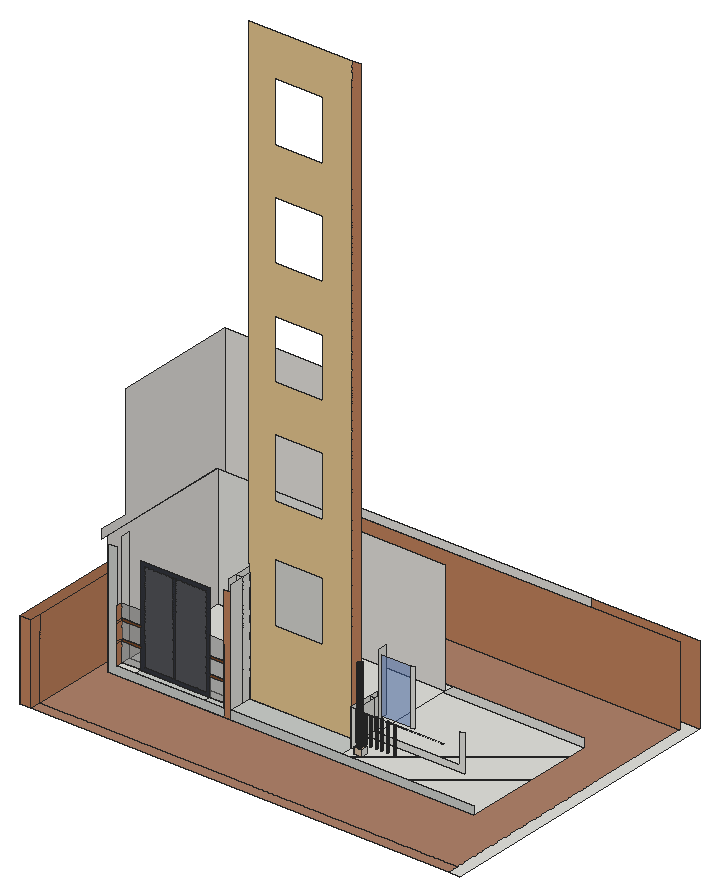
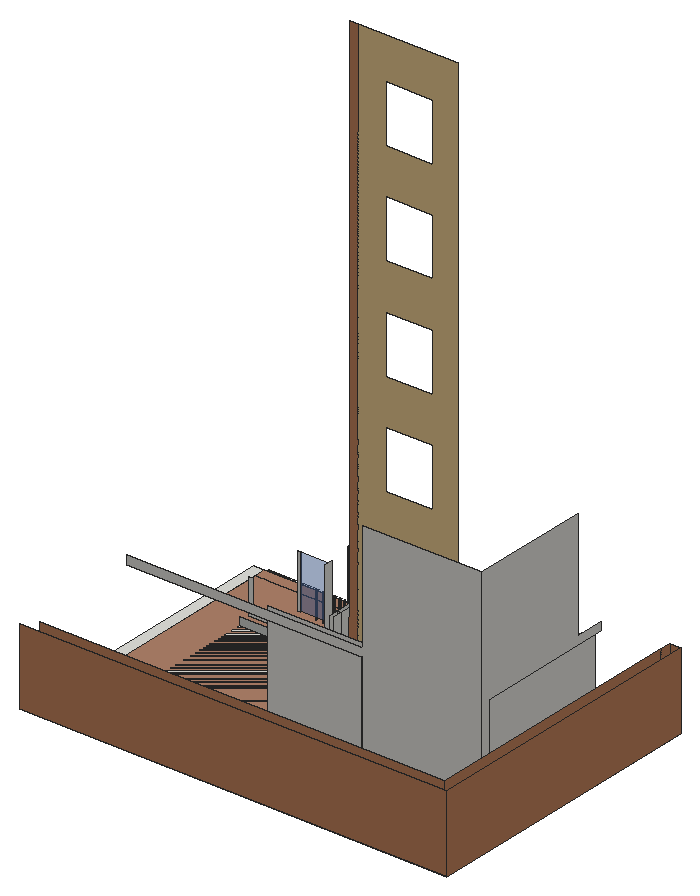
# SketchUp Ruby script. Lengths in inches.
U = 1.inch
M = Sketchup.active_model
def pt(a) = Geom::Point3d.new(a.map { |v| v * U })
def face(e, loops, mat)
  f = e.add_face(loops[0].map { |a| pt(a) })
  loops[1..].each { |l| e.add_face(l.map { |a| pt(a) }).erase! }
  f.material = f.back_material = mat if mat
  f
end
# faces: each face lists its corners as indices into pts; further lists are holes
def faces(e, pts, list, mat = nil) = list.each { |f| face(e, (f[0].is_a?(Array) ? f : [f]).map { |l| l.map { |i| pts[i] } }, mat) }
# xy, xz, yz: faces in a plane at the given z, y or x. An outline is a flat list of corners, or four numbers for a rectangle; further outlines are holes
def ring(l) = l.size == 4 ? [[l[0], l[1]], [l[2], l[1]], [l[2], l[3]], [l[0], l[3]]] : l.each_slice(2).to_a
def flat(e, list, mat, &to3) = list.each { |f| face(e, (f[0].is_a?(Array) ? f : [f]).map { |l| ring(l).map { |u, v| to3.(u, v) } }, mat) }
def xy(e, z, list, mat = nil) = flat(e, list, mat) { |x, y| [x, y, z] }
def xz(e, y, list, mat = nil) = flat(e, list, mat) { |x, z| [x, y, z] }
def yz(e, x, list, mat = nil) = flat(e, list, mat) { |y, z| [x, y, z] }
def lines(e, pts, list) = list.each { |a, b| e.add_line(pt(pts[a]), pt(pts[b])) }
# prism: a flat outline (further loops are holes) pulled along v
def prism(e, loops, v, mat = nil)
  f = face(e, loops, mat); d = Geom::Vector3d.new(v.map { |x| x * U })
  f.pushpull(f.normal.samedirection?(d) ? d.length : -d.length)
end
def box(e, o, s, mat = nil) = prism(e, [[o, [o[0] + s[0], o[1], o[2]], [o[0] + s[0], o[1] + s[1], o[2]], [o[0], o[1] + s[1], o[2]]]], [0, 0, s[2]], mat)
def at(x, y, z, deg = 0) = Geom::Transformation.translation(pt([x, y, z])) * Geom::Transformation.rotation(ORIGIN, Z_AXIS, deg.degrees)
def axes(o, x, y, z) = Geom::Transformation.new([*x, 0, *y, 0, *z, 0, *pt(o).to_a, 1])
def part(name) = M.definitions.add(name)
# library, detail: a bought-in or finely detailed component or shape, given as its bounding box
def library(name, o, s) = part(name).tap { |d| box(d.entities, o, s) }
def detail(e, o, s) = box(e.add_group.entities, o, s)
def put(e, d, t, mat = nil) = e.add_instance(d, t).tap { |i| i.material = mat if mat }
def group(e, t, mat = nil) = e.add_group.tap { |g| g.transformation = t; g.material = mat if mat }.entities
root = M.entities
M.materials.add("[Basic Tile]").color = [203, 206, 202]
M.materials.add("[Blinds Roman Hobbled Blue]").color = [81, 82, 87]
M.materials.add("[Formica Laminate Dark]").color = [50, 53, 60]
M.materials.add("[Formica Laminate Light]").color = [213, 189, 164]
M.materials.add("[Formica Speckled Grey]").color = [112, 125, 132]
M.materials.add("[Pavers Driveway Brick]").color = [176, 130, 106]
M.materials.add("[Stone Sandstone Ashlar Light]").color = [226, 196, 141]
M.materials.add("[Terrazzo Tile Accent]").color = [224, 221, 217]
M.materials.add("[Translucent Glass Blue]").color = [85, 126, 201]
M.materials["[Translucent Glass Blue]"].alpha = 0.5
M.materials.add("[Translucent Glass Gray]").color = [128, 128, 128]
M.materials["[Translucent Glass Gray]"].alpha = 0.5
M.materials.add("[Wood Veneer 01]").color = [120, 70, 37]
M.materials.add("[Wood Veneer 02]").color = [190, 128, 91]
xy(root,0,[[0,0,0,319.32,467.51,319.32,467.51,0,455.72,0,455.72,307.53,11.79,307.53,11.79,0],[22.54,88.35,411.85,235.11],[21.57,235.11,22.54,244.83],[22.54,235.11,153.36,244.83]])
xy(root,0,[[11.79,0,455.72,11.79],[[11.79,11.79,455.72,307.53],[21.57,235.11,22.54,244.83]]],"[Pavers Driveway Brick]")
xy(root,9,[[32.26,88.35,52.55,94.67],[32.26,94.67,146.55,104.39],[146.55,104.39,153.36,225.39],[153.36,114.1,271.94,225.39],[153.36,225.39,271.94,235.11]])
xy(root,9,[[52.55,88.35,126.05,94.67],[126.05,88.35,146.55,94.67],[153.36,88.35,271.94,114.1]],"[Basic Tile]")
xy(root,24.1875,[[296.1,73.57,304.9375,80.01]],"[Formica Laminate Light]")
xy(root,31.3,[[300.49,74.4375,299.88,74.44,299.3,74.61,298.78,74.92,298.36,75.35,298.0625,75.875,297.91,76.46,297.92,77.0625,298.09,77.64,298.39,78.16,298.82,78.58,299.35,78.88,299.9375,79.03,300.54,79.02,301.12,78.86,301.64,78.55,302.0625,78.12,302.36,77.59,302.51,77.01,302.5,76.4,302.34,75.82,302.03,75.3,301.6,74.88,301.07,74.59],[296.0625,81.89,295.89,81.92,295.72,81.98,295.58,82.09,295.47,82.24,295.4,82.4,295.375,82.58,295.4,82.76,295.47,82.92,295.58,83.07,295.72,83.18,295.89,83.24,296.0625,83.27,296.24,83.24,296.41,83.18,296.55,83.07,296.66,82.92,296.73,82.76,296.75,82.58,296.73,82.4,296.66,82.24,296.55,82.09,296.41,81.98,296.24,81.92],[307.125,81.89,306.95,81.92,306.78,81.98,306.64,82.09,306.53,82.24,306.46,82.4,306.4375,82.58,306.46,82.76,306.53,82.92,306.64,83.07,306.78,83.18,306.95,83.24,307.125,83.27,307.3,83.24,307.47,83.18,307.61,83.07,307.72,82.92,307.79,82.76,307.8125,82.58,307.79,82.4,307.72,82.24,307.61,82.09,307.47,81.98,307.3,81.92],[313.75,81.89,313.57,81.92,313.41,81.98,313.27,82.09,313.16,82.24,313.09,82.4,313.0625,82.58,313.09,82.76,313.16,82.92,313.27,83.07,313.41,83.18,313.57,83.24,313.75,83.27,313.93,83.24,314.1,83.18,314.24,83.07,314.35,82.92,314.42,82.76,314.4375,82.58,314.42,82.4,314.35,82.24,314.24,82.09,314.1,81.98,313.93,81.92],[318.5625,81.89,318.39,81.92,318.22,81.98,318.08,82.09,317.97,82.24,317.9,82.4,317.875,82.58,317.9,82.76,317.97,82.92,318.08,83.07,318.22,83.18,318.39,83.24,318.5625,83.27,318.74,83.24,318.91,83.18,319.05,83.07,319.16,82.92,319.23,82.76,319.25,82.58,319.23,82.4,319.16,82.24,319.05,82.09,318.91,81.98,318.74,81.92],
  [325.0625,81.89,324.89,81.92,324.72,81.98,324.58,82.09,324.47,82.24,324.4,82.4,324.375,82.58,324.4,82.76,324.47,82.92,324.58,83.07,324.72,83.18,324.89,83.24,325.0625,83.27,325.24,83.24,325.41,83.18,325.55,83.07,325.66,82.92,325.73,82.76,325.75,82.58,325.73,82.4,325.66,82.24,325.55,82.09,325.41,81.98,325.24,81.92],[332.6875,81.89,332.51,81.92,332.35,81.98,332.2,82.09,332.09,82.24,332.02,82.4,332,82.58,332.02,82.76,332.09,82.92,332.2,83.07,332.35,83.18,332.51,83.24,332.6875,83.27,332.87,83.24,333.03,83.18,333.18,83.07,333.28,82.92,333.35,82.76,333.375,82.58,333.35,82.4,333.28,82.24,333.18,82.09,333.03,81.98,332.87,81.92]])
xy(root,31.3,[[[296.1,73.57,304.9375,80.01],[300.49,74.4375,299.88,74.44,299.3,74.61,298.78,74.92,298.36,75.35,298.0625,75.875,297.91,76.46,297.92,77.0625,298.09,77.64,298.39,78.16,298.82,78.58,299.35,78.88,299.9375,79.03,300.54,79.02,301.12,78.86,301.64,78.55,302.0625,78.12,302.36,77.59,302.51,77.01,302.5,76.4,302.34,75.82,302.03,75.3,301.6,74.88,301.07,74.59]]],"[Formica Laminate Light]")
xy(root,60.24,[[296.0625,81.89,296.24,81.92,296.41,81.98,296.55,82.09,296.66,82.24,296.73,82.4,296.75,82.58,296.73,82.76,296.66,82.92,296.55,83.07,296.41,83.18,296.24,83.24,296.0625,83.27,295.89,83.24,295.72,83.18,295.58,83.07,295.47,82.92,295.4,82.76,295.375,82.58,295.4,82.4,295.47,82.24,295.58,82.09,295.72,81.98,295.89,81.92]])
xy(root,60.36,[[307.125,81.89,307.3,81.92,307.47,81.98,307.61,82.09,307.72,82.24,307.79,82.4,307.8125,82.58,307.79,82.76,307.72,82.92,307.61,83.07,307.47,83.18,307.3,83.24,307.125,83.27,306.95,83.24,306.78,83.18,306.64,83.07,306.53,82.92,306.46,82.76,306.4375,82.58,306.46,82.4,306.53,82.24,306.64,82.09,306.78,81.98,306.95,81.92],[332.6875,81.89,332.87,81.92,333.03,81.98,333.18,82.09,333.28,82.24,333.35,82.4,333.375,82.58,333.35,82.76,333.28,82.92,333.18,83.07,333.03,83.18,332.87,83.24,332.6875,83.27,332.51,83.24,332.35,83.18,332.2,83.07,332.09,82.92,332.02,82.76,332,82.58,332.02,82.4,332.09,82.24,332.2,82.09,332.35,81.98,332.51,81.92]])
xy(root,60.42,[[301.8125,81.89,301.99,81.92,302.16,81.98,302.3,82.09,302.41,82.24,302.48,82.4,302.5,82.58,302.48,82.76,302.41,82.92,302.3,83.07,302.16,83.18,301.99,83.24,301.8125,83.27,301.64,83.24,301.47,83.18,301.33,83.07,301.22,82.92,301.15,82.76,301.125,82.58,301.15,82.4,301.22,82.24,301.33,82.09,301.47,81.98,301.64,81.92]])
xy(root,60.86,[[318.5625,81.89,318.74,81.92,318.91,81.98,319.05,82.09,319.16,82.24,319.23,82.4,319.25,82.58,319.23,82.76,319.16,82.92,319.05,83.07,318.91,83.18,318.74,83.24,318.5625,83.27,318.39,83.24,318.22,83.18,318.08,83.07,317.97,82.92,317.9,82.76,317.875,82.58,317.9,82.4,317.97,82.24,318.08,82.09,318.22,81.98,318.39,81.92]])
xy(root,61.01,[[324.76,81.97,325.37,81.97,325.41,81.98,325.55,82.09,325.66,82.24,325.73,82.4,325.75,82.58,325.73,82.76,325.66,82.92,325.55,83.07,325.41,83.18,325.24,83.24,325.0625,83.27,324.89,83.24,324.72,83.18,324.58,83.07,324.47,82.92,324.4,82.76,324.375,82.58,324.4,82.4,324.47,82.24,324.58,82.09,324.72,81.98]])
xy(root,61.01,[[325.0625,81.89,325.24,81.92,325.37,81.97,324.76,81.97,324.89,81.92]],"[Formica Laminate Dark]")
xy(root,61.11,[[313.75,81.89,313.93,81.92,314.1,81.98,314.24,82.09,314.35,82.24,314.42,82.4,314.4375,82.58,314.42,82.76,314.35,82.92,314.24,83.07,314.1,83.18,313.93,83.24,313.75,83.27,313.57,83.24,313.41,83.18,313.27,83.07,313.16,82.92,313.09,82.76,313.0625,82.58,313.09,82.4,313.16,82.24,313.27,82.09,313.41,81.98,313.57,81.92]],"[Formica Laminate Dark]")
xz(root,0,[[0,0,11.79,84]],"[Wood Veneer 02]")
xz(root,73.57,[[296.1,24.1875,304.9375,31.3]],"[Formica Laminate Light]")
xz(root,80.01,[[288.3125,24.1875,296.1,24.1875,296.1,31.3,293.16,31.3,293.16,63.125,288.3125,63.125],[296.1,24.1875,304.9375,31.3]])
xz(root,88.35,[[22.54,0,146.55,0,146.55,9,32.26,9,32.26,121.75,22.54,121.75],[153.36,0,411.85,9]],"[Basic Tile]")
xz(root,88.35,[[146.55,0,153.36,121.75]],"[Wood Veneer 02]")
xz(root,94.67,[[56.79,13.23,86.91,109.13],[90.25,13.23,121.82,109.13]],"[Blinds Roman Hobbled Blue]")
xz(root,94.67,[[[52.55,9,126.05,113.36],[56.79,13.23,121.82,109.13]],[86.91,13.23,90.25,109.13]],"[Formica Laminate Dark]")
xz(root,94.67,[[32.26,9,52.55,29.84],[126.05,9,146.55,28.84],[126.05,31.25,146.55,46.22],[32.26,32.25,52.55,49.24],[126.05,48.63,146.55,68.52],
  [32.26,51.65,52.55,66.22]],"[Translucent Glass Gray]")
xz(root,94.67,[[126.05,28.84,146.55,31.25],[32.26,29.84,52.55,32.25],[126.05,46.22,146.55,48.63],[32.26,49.24,52.55,51.65]],"[Wood Veneer 01]")
xz(root,104.39,[[146.55,9,153.36,129],[288.3125,24.1875,288.3125,63.125,293.16,63.125,293.16,31.3,384.76,31.3,384.76,63.125,389.375,63.125,389.375,24.1875],[332.63,48.23,335.97,107.2]])
xz(root,104.39,[[301.61,48.23,332.63,107.2]],"[Translucent Glass Blue]")
xz(root,114.1,[[[153.36,9,261.97,9,261.97,654.5625,152.39,654.5625,152.39,138,153.36,138],[179.41,545.4375,230.79,609.125],[179.41,87.4375,230.79,151.125],[179.41,432.625,230.79,496.3125],[179.41,206.5625,230.79,270.25],[179.41,319.3125,230.79,383]]],"[Stone Sandstone Ashlar Light]")
xz(root,114.1,[[261.97,9,271.94,9,270.97,129,270.97,654.5625,261.97,654.5625]],"[Wood Veneer 02]")
xz(root,225.39,[[146.55,9,153.36,129]])
xz(root,225.39,[[153.36,9,271.94,129]],"[Terrazzo Tile Accent]")
xz(root,235.11,[[21.57,0,22.54,129],[22.54,0,153.36,129],[153.36,0,411.85,9]])
xz(root,244.83,[[21.57,0,21.57,258,152.39,258,152.39,138,410.88,138,410.88,129,153.36,129,153.36,0]],"[Terrazzo Tile Accent]")
xz(root,307.53,[[11.79,0,455.72,84]],"[Wood Veneer 02]")
xz(root,319.32,[[0,0,467.51,84]],"[Wood Veneer 02]")
yz(root,0,[[0,0,319.32,84]],"[Wood Veneer 02]")
yz(root,11.79,[[0,0,11.79,84],[11.79,0,307.53,84]],"[Wood Veneer 02]")
yz(root,21.57,[[235.11,0,235.11,129,82.1,129,82.1,138,114.1,138,114.1,258,244.83,258,244.83,0]],"[Terrazzo Tile Accent]")
yz(root,22.54,[[88.35,0,235.11,129]],"[Terrazzo Tile Accent]")
yz(root,32.26,[[94.67,9,104.39,129]])
yz(root,32.26,[[88.35,9,94.67,29.84],[88.35,29.84,94.67,32.25],[88.35,32.25,94.67,49.24],[88.35,49.24,94.67,51.65],[88.35,51.65,94.67,66.22]],"[Wood Veneer 02]")
yz(root,146.55,[[94.67,9,104.39,129],[104.39,9,225.39,129]])
yz(root,146.55,[[88.35,9,94.67,28.84],[88.35,28.84,94.67,31.25],[88.35,31.25,94.67,46.22],[88.35,46.22,94.67,48.63],[88.35,48.63,94.67,68.52]],"[Wood Veneer 02]")
yz(root,153.36,[[235.11,0,244.83,129],[88.35,9,104.39,129],[104.39,9,114.1,129],[114.1,9,225.39,129],[225.39,9,235.11,129]])
yz(root,288.3125,[[80.01,24.1875,104.39,63.125],[104.39,24.1875,114.1,63.125]])
yz(root,293.16,[[[80.01,31.3,104.39,62.16],[82.67,59.79,82.46,59.82,82.26,59.9,82.1,60.03,81.97,60.2,81.89,60.39,81.86,60.6,81.89,60.8125,81.97,61.01,82.1,61.18,82.26,61.31,82.46,61.39,82.67,61.42,82.88,61.39,83.08,61.31,83.25,61.18,83.375,61.01,83.46,60.8125,83.48,60.6,83.46,60.39,83.375,60.2,83.25,60.03,83.08,59.9,82.88,59.82]],[104.39,31.3,114.1,62.16]])
yz(root,296.1,[[73.57,24.1875,80.01,31.3]],"[Formica Laminate Light]")
yz(root,298,[[104.39,44.62,114.1,110.81]])
yz(root,304.9375,[[73.57,24.1875,80.01,31.3]])
p = [[299.3,74.61,31.3],[299.88,74.44,31.3],[299.88,74.44,110.81],[299.3,74.61,110.81],[300.49,74.4375,31.3],[300.49,74.4375,110.81],
  [301.07,74.59,31.3],[301.07,74.59,110.81],[298.78,74.92,31.3],[298.78,74.92,110.81],[301.6,74.88,31.3],[301.6,74.88,110.81],
  [298.36,75.35,31.3],[298.36,75.35,110.81],[302.03,75.3,31.3],[302.03,75.3,110.81],[298.0625,75.875,31.3],[298.0625,75.875,110.81],
  [302.34,75.82,31.3],[302.34,75.82,110.81],[302.5,76.4,31.3],[302.5,76.4,110.81],[297.91,76.46,31.3],[297.91,76.46,110.81],
  [302.51,77.01,31.3],[302.51,77.01,110.81],[297.92,77.0625,31.3],[297.92,77.0625,110.81],[302.36,77.59,31.3],[302.36,77.59,110.81],
  [298.09,77.64,31.3],[298.09,77.64,110.81],[298.39,78.16,31.3],[298.39,78.16,110.81],[302.0625,78.12,31.3],[302.0625,78.12,110.81],
  [301.64,78.55,31.3],[301.64,78.55,110.81],[298.82,78.58,31.3],[298.82,78.58,110.81],[299.35,78.88,31.3],[299.35,78.88,110.81],
  [301.12,78.86,31.3],[301.12,78.86,110.81],[299.9375,79.03,31.3],[299.9375,79.03,110.81],[300.54,79.02,31.3],[300.54,79.02,110.81],
  [295.72,81.98,31.3],[295.89,81.92,31.3],[295.89,81.92,60.24],[295.72,81.98,60.24],[296.0625,81.89,31.3],[296.0625,81.89,60.24],
  [296.24,81.92,31.3],[296.24,81.92,60.24],[296.41,81.98,31.3],[296.41,81.98,60.24],[301.47,81.98,31.3],[301.64,81.92,31.3],
  [301.64,81.92,60.42],[301.47,81.98,60.42],[301.8125,81.89,31.3],[301.8125,81.89,60.42],[301.99,81.92,31.3],[301.99,81.92,60.42],
  [302.16,81.98,31.3],[302.16,81.98,60.42],[306.78,81.98,31.3],[306.95,81.92,31.3],[306.95,81.92,60.36],[306.78,81.98,60.36],
  [307.125,81.89,31.3],[307.125,81.89,60.36],[307.3,81.92,31.3],[307.3,81.92,60.36],[307.47,81.98,31.3],[307.47,81.98,60.36],
  [313.41,81.98,31.3],[313.57,81.92,31.3],[313.57,81.92,61.11],[313.41,81.98,61.11],[313.75,81.89,31.3],[313.75,81.89,61.11],
  [313.93,81.92,31.3],[313.93,81.92,61.11],[314.1,81.98,31.3],[314.1,81.98,61.11],[318.22,81.98,31.3],[318.39,81.92,31.3],
  [318.39,81.92,60.86],[318.22,81.98,60.86],[318.5625,81.89,31.3],[318.5625,81.89,60.86],[318.74,81.92,31.3],[318.74,81.92,60.86],
  [318.91,81.98,31.3],[318.91,81.98,60.86],[324.72,81.98,31.3],[324.89,81.92,31.3],[324.89,81.92,61.01],[324.76,81.97,61.01],
  [324.72,81.98,61.01],[325.0625,81.89,31.3],[325.0625,81.89,61.01],[325.24,81.92,31.3],[325.24,81.92,61.01],[325.41,81.98,31.3],
  [325.41,81.98,61.01],[325.37,81.97,61.01],[332.35,81.98,31.3],[332.51,81.92,31.3],[332.51,81.92,60.36],[332.35,81.98,60.36],
  [332.6875,81.89,31.3],[332.6875,81.89,60.36],[332.87,81.92,31.3],[332.87,81.92,60.36],[333.03,81.98,31.3],[333.03,81.98,60.36],
  [295.58,82.09,31.3],[295.58,82.09,60.24],[296.55,82.09,31.3],[296.55,82.09,60.24],[301.33,82.09,31.3],[301.33,82.09,60.42],
  [302.3,82.09,31.3],[302.3,82.09,60.42],[306.64,82.09,31.3],[306.64,82.09,60.36],[307.61,82.09,31.3],[307.61,82.09,60.36],
  [313.27,82.09,31.3],[313.27,82.09,61.11],[314.24,82.09,31.3],[314.24,82.09,61.11],[318.08,82.09,31.3],[318.08,82.09,60.86],
  [319.05,82.09,31.3],[319.05,82.09,60.86],[324.58,82.09,31.3],[324.58,82.09,61.01],[325.55,82.09,31.3],[325.55,82.09,61.01],
  [332.2,82.09,31.3],[332.2,82.09,60.36],[333.18,82.09,31.3],[333.18,82.09,60.36],[295.47,82.24,31.3],[295.47,82.24,60.24],
  [296.66,82.24,31.3],[296.66,82.24,60.24],[301.22,82.24,31.3],[301.22,82.24,60.42],[302.41,82.24,31.3],[302.41,82.24,60.42],
  [306.53,82.24,31.3],[306.53,82.24,60.36],[307.72,82.24,31.3],[307.72,82.24,60.36],[313.16,82.24,31.3],[313.16,82.24,61.11],
  [314.35,82.24,31.3],[314.35,82.24,61.11],[317.97,82.24,31.3],[317.97,82.24,60.86],[319.16,82.24,31.3],[319.16,82.24,60.86],
  [324.47,82.24,31.3],[324.47,82.24,61.01],[325.66,82.24,31.3],[325.66,82.24,61.01],[332.09,82.24,31.3],[332.09,82.24,60.36],
  [333.28,82.24,31.3],[333.28,82.24,60.36],[295.4,82.4,31.3],[295.4,82.4,60.24],[296.73,82.4,31.3],[296.73,82.4,60.24],
  [301.15,82.4,31.3],[301.15,82.4,60.42],[302.48,82.4,31.3],[302.48,82.4,60.42],[306.46,82.4,31.3],[306.46,82.4,60.36],
  [307.79,82.4,31.3],[307.79,82.4,60.36],[313.09,82.4,31.3],[313.09,82.4,61.11],[314.42,82.4,31.3],[314.42,82.4,61.11],
  [317.9,82.4,31.3],[317.9,82.4,60.86],[319.23,82.4,31.3],[319.23,82.4,60.86],[324.4,82.4,31.3],[324.4,82.4,61.01],
  [325.73,82.4,31.3],[325.73,82.4,61.01],[332.02,82.4,31.3],[332.02,82.4,60.36],[333.35,82.4,31.3],[333.35,82.4,60.36],
  [295.375,82.58,31.3],[295.375,82.58,60.24],[296.75,82.58,31.3],[296.75,82.58,60.24],[301.125,82.58,31.3],[301.125,82.58,60.42],
  [302.5,82.58,31.3],[302.5,82.58,60.42],[306.4375,82.58,31.3],[306.4375,82.58,60.36],[307.8125,82.58,31.3],[307.8125,82.58,60.36],
  [313.0625,82.58,31.3],[313.0625,82.58,61.11],[314.4375,82.58,31.3],[314.4375,82.58,61.11],[317.875,82.58,31.3],[317.875,82.58,60.86],
  [319.25,82.58,31.3],[319.25,82.58,60.86],[324.375,82.58,31.3],[324.375,82.58,61.01],[325.75,82.58,31.3],[325.75,82.58,61.01],
  [332,82.58,31.3],[332,82.58,60.36],[333.375,82.58,31.3],[333.375,82.58,60.36],[295.4,82.76,31.3],[295.4,82.76,60.24],
  [296.73,82.76,31.3],[296.73,82.76,60.24],[301.15,82.76,31.3],[301.15,82.76,60.42],[302.48,82.76,31.3],[302.48,82.76,60.42],
  [306.46,82.76,31.3],[306.46,82.76,60.36],[307.79,82.76,31.3],[307.79,82.76,60.36],[313.09,82.76,31.3],[313.09,82.76,61.11],
  [314.42,82.76,31.3],[314.42,82.76,61.11],[317.9,82.76,31.3],[317.9,82.76,60.86],[319.23,82.76,31.3],[319.23,82.76,60.86],
  [324.4,82.76,31.3],[324.4,82.76,61.01],[325.73,82.76,31.3],[325.73,82.76,61.01],[332.02,82.76,31.3],[332.02,82.76,60.36],
  [333.35,82.76,31.3],[333.35,82.76,60.36],[295.47,82.92,31.3],[295.47,82.92,60.24],[296.66,82.92,31.3],[296.66,82.92,60.24],
  [301.22,82.92,31.3],[301.22,82.92,60.42],[302.41,82.92,31.3],[302.41,82.92,60.42],[306.53,82.92,31.3],[306.53,82.92,60.36],
  [307.72,82.92,31.3],[307.72,82.92,60.36],[313.16,82.92,31.3],[313.16,82.92,61.11],[314.35,82.92,31.3],[314.35,82.92,61.11],
  [317.97,82.92,31.3],[317.97,82.92,60.86],[319.16,82.92,31.3],[319.16,82.92,60.86],[324.47,82.92,31.3],[324.47,82.92,61.01],
  [325.66,82.92,31.3],[325.66,82.92,61.01],[332.09,82.92,31.3],[332.09,82.92,60.36],[333.28,82.92,31.3],[333.28,82.92,60.36],
  [295.58,83.07,31.3],[295.58,83.07,60.24],[296.55,83.07,31.3],[296.55,83.07,60.24],[301.33,83.07,31.3],[301.33,83.07,60.42],
  [302.3,83.07,31.3],[302.3,83.07,60.42],[306.64,83.07,31.3],[306.64,83.07,60.36],[307.61,83.07,31.3],[307.61,83.07,60.36],
  [313.27,83.07,31.3],[313.27,83.07,61.11],[314.24,83.07,31.3],[314.24,83.07,61.11],[318.08,83.07,31.3],[318.08,83.07,60.86],
  [319.05,83.07,31.3],[319.05,83.07,60.86],[324.58,83.07,31.3],[324.58,83.07,61.01],[325.55,83.07,31.3],[325.55,83.07,61.01],
  [332.2,83.07,31.3],[332.2,83.07,60.36],[333.18,83.07,31.3],[333.18,83.07,60.36],[295.72,83.18,31.3],[295.72,83.18,60.24],
  [296.41,83.18,31.3],[296.41,83.18,60.24],[301.47,83.18,31.3],[301.47,83.18,60.42],[302.16,83.18,31.3],[302.16,83.18,60.42],
  [306.78,83.18,31.3],[306.78,83.18,60.36],[307.47,83.18,31.3],[307.47,83.18,60.36],[313.41,83.18,31.3],[313.41,83.18,61.11],
  [314.1,83.18,31.3],[314.1,83.18,61.11],[318.22,83.18,31.3],[318.22,83.18,60.86],[318.91,83.18,31.3],[318.91,83.18,60.86],
  [324.72,83.18,31.3],[324.72,83.18,61.01],[325.41,83.18,31.3],[325.41,83.18,61.01],[332.35,83.18,31.3],[332.35,83.18,60.36],
  [333.03,83.18,31.3],[333.03,83.18,60.36],[295.89,83.24,31.3],[295.89,83.24,60.24],[296.0625,83.27,31.3],[296.0625,83.27,60.24],
  [296.24,83.24,31.3],[296.24,83.24,60.24],[301.64,83.24,31.3],[301.64,83.24,60.42],[301.8125,83.27,31.3],[301.8125,83.27,60.42],
  [301.99,83.24,31.3],[301.99,83.24,60.42],[306.95,83.24,31.3],[306.95,83.24,60.36],[307.125,83.27,31.3],[307.125,83.27,60.36],
  [307.3,83.24,31.3],[307.3,83.24,60.36],[313.57,83.24,31.3],[313.57,83.24,61.11],[313.75,83.27,31.3],[313.75,83.27,61.11],
  [313.93,83.24,31.3],[313.93,83.24,61.11],[318.39,83.24,31.3],[318.39,83.24,60.86],[318.5625,83.27,31.3],[318.5625,83.27,60.86],
  [318.74,83.24,31.3],[318.74,83.24,60.86],[324.89,83.24,31.3],[324.89,83.24,61.01],[325.0625,83.27,31.3],[325.0625,83.27,61.01],
  [325.24,83.24,31.3],[325.24,83.24,61.01],[332.51,83.24,31.3],[332.51,83.24,60.36],[332.6875,83.27,31.3],[332.6875,83.27,60.36],
  [332.87,83.24,31.3],[332.87,83.24,60.36],[384.76,81.89,60.8125],[384.76,81.97,61.01],[293.16,81.97,61.01],[293.16,81.89,60.8125]]
faces(root,p,[[0,1,2,3],[1,4,5,2],[4,6,7,5],[8,0,3,9],[6,10,11,7],[12,8,9,13],[10,14,15,11],[16,12,13,17],
  [14,18,19,15],[18,20,21,19],[22,16,17,23],[20,24,25,21],[26,22,23,27],[24,28,29,25],[30,26,27,31],[32,30,31,33],
  [28,34,35,29],[34,36,37,35],[38,32,33,39],[40,38,39,41],[36,42,43,37],[44,40,41,45],[42,46,47,43],[46,44,45,47]],"[Formica Speckled Grey]")
faces(root,p,[[48,49,50,51],[49,52,53,50],[52,54,55,53],[54,56,57,55],[58,59,60,61],[59,62,63,60],[62,64,65,63],[64,66,67,65],
  [68,69,70,71],[69,72,73,70],[72,74,75,73],[74,76,77,75],[78,79,80,81],[79,82,83,80],[82,84,85,83],[84,86,87,85],
  [88,89,90,91],[89,92,93,90],[92,94,95,93],[94,96,97,95],[98,99,100,101,102],[99,103,104,100],[103,105,106,104],[105,107,108,109,106],
  [110,111,112,113],[111,114,115,112],[114,116,117,115],[116,118,119,117],[120,48,51,121],[56,122,123,57],[124,58,61,125],[66,126,127,67],
  [128,68,71,129],[76,130,131,77],[132,78,81,133],[86,134,135,87],[136,88,91,137],[96,138,139,97],[140,98,102,141],[107,142,143,108],
  [144,110,113,145],[118,146,147,119],[148,120,121,149],[122,150,151,123],[152,124,125,153],[126,154,155,127],[156,128,129,157],[130,158,159,131],
  [160,132,133,161],[134,162,163,135],[164,136,137,165],[138,166,167,139],[168,140,141,169],[142,170,171,143],[172,144,145,173],[146,174,175,147],
  [176,148,149,177],[150,178,179,151],[180,152,153,181],[154,182,183,155],[184,156,157,185],[158,186,187,159],[188,160,161,189],[162,190,191,163],
  [192,164,165,193],[166,194,195,167],[196,168,169,197],[170,198,199,171],[200,172,173,201],[174,202,203,175],[204,176,177,205],[178,206,207,179],
  [208,180,181,209],[182,210,211,183],[212,184,185,213],[186,214,215,187],[216,188,189,217],[190,218,219,191],[220,192,193,221],[194,222,223,195],
  [224,196,197,225],[198,226,227,199],[228,200,201,229],[202,230,231,203],[232,204,205,233],[206,234,235,207],[236,208,209,237],[210,238,239,211],
  [240,212,213,241],[214,242,243,215],[244,216,217,245],[218,246,247,219],[248,220,221,249],[222,250,251,223],[252,224,225,253],[226,254,255,227],
  [256,228,229,257],[230,258,259,231],[260,232,233,261],[234,262,263,235],[264,236,237,265],[238,266,267,239],[268,240,241,269],[242,270,271,243],
  [272,244,245,273],[246,274,275,247],[276,248,249,277],[250,278,279,251],[280,252,253,281],[254,282,283,255],[284,256,257,285],[258,286,287,259],
  [288,260,261,289],[262,290,291,263],[292,264,265,293],[266,294,295,267],[296,268,269,297],[270,298,299,271],[300,272,273,301],[274,302,303,275],
  [304,276,277,305],[278,306,307,279],[308,280,281,309],[282,310,311,283],[312,284,285,313],[286,314,315,287],[316,288,289,317],[290,318,319,291],
  [320,292,293,321],[294,322,323,295],[324,296,297,325],[298,326,327,299],[328,300,301,329],[302,330,331,303],[332,304,305,333],[306,334,335,307],
  [336,308,309,337],[310,338,339,311],[340,312,313,341],[314,342,343,315],[344,316,317,345],[346,344,345,347],[348,346,347,349],[318,348,349,319],
  [350,320,321,351],[352,350,351,353],[354,352,353,355],[322,354,355,323],[356,324,325,357],[358,356,357,359],[360,358,359,361],[326,360,361,327],
  [362,328,329,363],[364,362,363,365],[366,364,365,367],[330,366,367,331],[368,332,333,369],[370,368,369,371],[372,370,371,373],[334,372,373,335],
  [374,336,337,375],[376,374,375,377],[378,376,377,379],[338,378,379,339],[380,340,341,381],[382,380,381,383],[384,382,383,385],[342,384,385,343],
  [386,387,109,101,388,389]],"[Formica Laminate Dark]")
